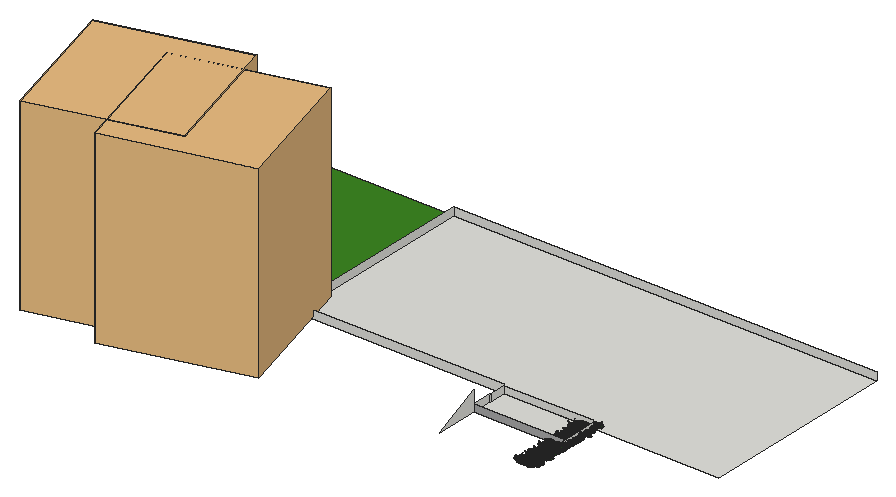
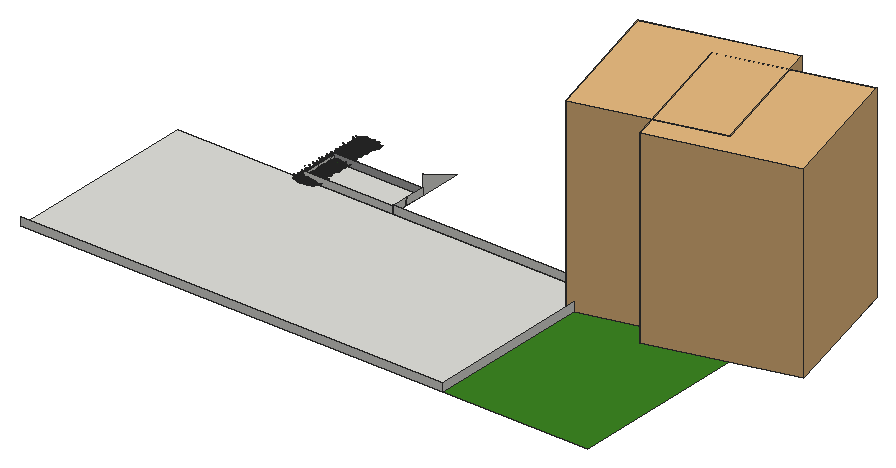
# SketchUp Ruby script. Lengths in inches.
U = 1.inch
M = Sketchup.active_model
def pt(a) = Geom::Point3d.new(a.map { |v| v * U })
def face(e, loops, mat)
  f = e.add_face(loops[0].map { |a| pt(a) })
  loops[1..].each { |l| e.add_face(l.map { |a| pt(a) }).erase! }
  f.material = f.back_material = mat if mat
  f
end
# faces: each face lists its corners as indices into pts; further lists are holes
def faces(e, pts, list, mat = nil) = list.each { |f| face(e, (f[0].is_a?(Array) ? f : [f]).map { |l| l.map { |i| pts[i] } }, mat) }
# xy, xz, yz: faces in a plane at the given z, y or x. An outline is a flat list of corners, or four numbers for a rectangle; further outlines are holes
def ring(l) = l.size == 4 ? [[l[0], l[1]], [l[2], l[1]], [l[2], l[3]], [l[0], l[3]]] : l.each_slice(2).to_a
def flat(e, list, mat, &to3) = list.each { |f| face(e, (f[0].is_a?(Array) ? f : [f]).map { |l| ring(l).map { |u, v| to3.(u, v) } }, mat) }
def xy(e, z, list, mat = nil) = flat(e, list, mat) { |x, y| [x, y, z] }
def xz(e, y, list, mat = nil) = flat(e, list, mat) { |x, z| [x, y, z] }
def yz(e, x, list, mat = nil) = flat(e, list, mat) { |y, z| [x, y, z] }
def lines(e, pts, list) = list.each { |a, b| e.add_line(pt(pts[a]), pt(pts[b])) }
# prism: a flat outline (further loops are holes) pulled along v
def prism(e, loops, v, mat = nil)
  f = face(e, loops, mat); d = Geom::Vector3d.new(v.map { |x| x * U })
  f.pushpull(f.normal.samedirection?(d) ? d.length : -d.length)
end
def box(e, o, s, mat = nil) = prism(e, [[o, [o[0] + s[0], o[1], o[2]], [o[0] + s[0], o[1] + s[1], o[2]], [o[0], o[1] + s[1], o[2]]]], [0, 0, s[2]], mat)
def at(x, y, z, deg = 0) = Geom::Transformation.translation(pt([x, y, z])) * Geom::Transformation.rotation(ORIGIN, Z_AXIS, deg.degrees)
def axes(o, x, y, z) = Geom::Transformation.new([*x, 0, *y, 0, *z, 0, *pt(o).to_a, 1])
def part(name) = M.definitions.add(name)
# library, detail: a bought-in or finely detailed component or shape, given as its bounding box
def library(name, o, s) = part(name).tap { |d| box(d.entities, o, s) }
def detail(e, o, s) = box(e.add_group.entities, o, s)
def put(e, d, t, mat = nil) = e.add_instance(d, t).tap { |i| i.material = mat if mat }
def group(e, t, mat = nil) = e.add_group.tap { |g| g.transformation = t; g.material = mat if mat }.entities
root = M.entities
M.materials.add("Material82").color = [68, 110, 58]
M.materials.add("Material83").color = [48, 90, 38]
M.materials.add("Material84").color = [68, 110, 48]
M.materials.add("Material85").color = [48, 90, 48]
M.materials.add("Material86").color = [58, 110, 58]
M.materials.add("Material87").color = [58, 90, 38]
M.materials.add("Material88").color = [68, 100, 58]
M.materials.add("Material89").color = [48, 100, 38]
M.materials.add("[Color M01]").color = [60, 133, 34]
M.materials.add("[Color M03]1").color = [170, 170, 170]
c1 = library("Palm tree",[-4.09,-4.52,0],[193.52,193.51,258.93])
c2 = part("Palm+Tree")
put(c2.entities,c1,at(25.51,-21.81,0,15))
c3 = library("Group\#612",[0,0,0],[32.91,53.52,103.45])
c4 = part("grass00")
p = [[-0.6875,0.15,0],[-0.56,0.08,5.52],[-0.04,0.03,2.76],[0.48,-0.02,0],[0.35,-0.02,5.52],[-0.1,-0.14,5.52],
  [-0.12,0.65,8.37],[-0.42,0.65,8.37]]
faces(c4.entities,p,[[0,1,2,3],[3,2,4],[1,5,2],[5,4,2],[1,6,5],[4,5,6],[7,6,1]])
c5 = part("Group16\#1")
put(c5.entities,c4,axes([1.44,-0.61,-0.01],[0.05352,0.12609,0],[-0.10704,0.04543,0.07239],[0.06664,-0.02828,0.11628]),"Material85")
put(c5.entities,c4,axes([0.76,-0.15,-0.01],[0.04676,0.24062,0],[-0.23162,0.04501,0.06642],[0.0652,-0.01267,0.23595]),"Material82")
put(c5.entities,c4,axes([0.79,0.01,-0.01],[-0.00606,0.34651,0],[-0.34381,-0.00602,0.0432],[0.04319,0.00076,0.34386]))
put(c5.entities,c4,axes([1,0.23,-0.01],[-0.07192,0.31144,0],[-0.28722,-0.06632,0.1236],[0.12043,0.02781,0.29478]),"Material84")
put(c5.entities,c4,axes([1.66,0.77,-0.01],[-0.13828,0.29651,0],[-0.21551,-0.1005,0.22471],[0.20365,0.09498,0.23779]),"Material89")
put(c5.entities,c4,axes([0.6875,0.52,-0.01],[-0.18126,0.24051,0],[-0.22746,-0.17142,0.09788],[0.07817,0.05891,0.28481]),"Material84")
put(c5.entities,c4,axes([0.68,0.78,-0.01],[-0.215,0.18688,0],[-0.12385,-0.14248,0.21334],[0.13995,0.16101,0.18878]),"Material82")
put(c5.entities,c4,axes([0.56,1,-0.01],[-0.13756,0.07624,0],[-0.06159,-0.11112,0.0927],[0.04494,0.08108,0.12705]),"Material84")
put(c5.entities,c4,axes([0.2,0.64,-0.01],[-0.23729,0.07254,0],[-0.05711,-0.18681,0.153],[0.04473,0.14632,0.19535]),"Material89")
put(c5.entities,c4,axes([0.0625,0.72,-0.01],[-0.28874,0.02525,0],[-0.02179,-0.24916,0.14647],[0.01276,0.14591,0.25012]),"Material82")
put(c5.entities,c4,axes([-0.08,0.62,-0.01],[-0.34089,-0.04187,0],[0.03255,-0.26504,0.216],[-0.02633,0.21439,0.26703]),"Material89")
put(c5.entities,c4,axes([-0.34,0.98,-0.01],[-0.14314,-0.0493,0],[0.04397,-0.12769,0.06843],[-0.02228,0.0647,0.13505]),"Material89")
put(c5.entities,c4,axes([-0.87,1.45,-0.01],[-0.23488,-0.14114,0],[0.13761,-0.22901,0.06087],[-0.03135,0.05217,0.26717]))
put(c5.entities,c4,axes([-0.72,0.77,-0.01],[-0.14208,-0.13251,0],[0.07209,-0.0773,0.16301],[-0.11118,0.11922,0.1057]),"Material89")
put(c5.entities,c4,axes([-0.62,0.43,-0.01],[-0.14845,-0.21203,0],[0.18654,-0.13061,0.12304],[-0.10079,0.07057,0.22772]),"Material82")
put(c5.entities,c4,axes([-0.68,0.29,-0.01],[-0.13639,-0.32136,0],[0.31723,-0.13464,0.05579],[-0.05136,0.0218,0.34462]),"Material83")
put(c5.entities,c4,axes([-0.64,0.125,-0.01],[-0.0458,-0.23569,0],[0.22124,-0.043,0.08276],[-0.08124,0.01579,0.22538]),"Material86")
put(c5.entities,c4,axes([-1.6,-0.03,-0.01],[0.00576,-0.32897,0],[0.27526,0.00482,0.18018],[-0.18015,-0.00315,0.2753]),"Material84")
put(c5.entities,c4,axes([-1.36,-0.31,-0.01],[0.05718,-0.24765,0],[0.18172,0.04196,0.17267],[-0.16825,-0.03885,0.1865]),"Material89")
put(c5.entities,c4,axes([-1.54,-0.72,-0.01],[0.06537,-0.14017,0],[0.13555,0.06321,0.03939],[-0.0357,-0.01665,0.14956]))
put(c5.entities,c4,axes([-1.19,-0.9,-0.01],[0.09597,-0.12735,0],[0.11214,0.08451,0.07557],[-0.06035,-0.04548,0.14042]),"Material88")
put(c5.entities,c4,axes([-0.47,-0.54,-0.01],[0.11588,-0.10072,0],[0.0618,0.0711,0.12124],[-0.07953,-0.0915,0.0942]))
put(c5.entities,c4,axes([-0.47,-0.84,-0.01],[0.11927,-0.0661,0],[0.06603,0.11913,0.00646],[-0.00313,-0.00565,0.13621]),"Material84")
put(c5.entities,c4,axes([-0.38,-1.24,-0.01],[0.28037,-0.08571,0],[0.0618,0.20215,0.20315],[-0.05939,-0.19428,0.21139]),"Material88")
put(c5.entities,c4,axes([-0.06,-0.66,-0.01],[0.22719,-0.01987,0],[0.01247,0.14255,0.17758],[-0.01547,-0.17691,0.1431]),"Material87")
put(c5.entities,c4,axes([0.11,-0.89,-0.01],[0.14882,0.01828,0],[-0.01058,0.08611,0.12229],[0.01491,-0.12138,0.08676]),"Material85")
put(c5.entities,c4,axes([0.25,-0.72,-0.01],[0.20481,0.07053,0],[-0.06206,0.18022,0.10291],[0.03351,-0.0973,0.1906]),"Material85")
put(c5.entities,c4,axes([0.85,-1.42,-0.01],[0.16481,0.09904,0],[-0.09472,0.15762,0.05616],[0.02893,-0.04814,0.18389]),"Material84")
put(c5.entities,c4,axes([1.01,-1.09,-0.01],[0.21858,0.20385,0],[-0.17495,0.1876,0.15339],[0.10462,-0.11218,0.25652]),"Material89")
put(c5.entities,c4,axes([1.01,-0.71,-0.01],[0.08733,0.12473,0],[-0.06445,0.04512,0.13037],[0.1068,-0.07477,0.07867]),"Material85")
c6 = part("Group15\#1")
put(c6.entities,c5,at(0,0,0))
c7 = part("3darcstudiotree_grass00\#1")
put(c7.entities,c6,at(0,0,0))
xy(root,-29.74,[[1163.9375,932.5,1248,932.62],[1534.38,994.94,1657.0625,1046.93],[1248,1046.93,1830.75,1318.18]])
xy(root,-29.74,[[1048.3125,932.62,1248,1318.18]],"[Color M01]")
xz(root,994.94,[[1534.38,-29.74,1657.0625,-19.8125]],"[Color M03]1")
xz(root,1046.93,[[1248,-29.74,1256.88,-19.8125],[1256.88,-29.74,1534.38,-18.36],[1534.38,-29.74,1657.0625,-19.8125]])
xz(root,1318.18,[[1248,-29.74,1830.75,-18.36]])
yz(root,1248,[[935.62,-29.74,994.94,-2.1875,994.94,-29.74],[994.94,-29.74,1046.93,-19.8125],[1046.93,-29.74,1318.18,-18.36]])
yz(root,1534.38,[[935.62,-29.74,994.94,-29.74,994.94,-2.1875],[994.94,-29.74,1022.06,-19.8125],[1022.06,-29.74,1023.55,-19.8125],[1023.55,-29.74,1046.93,-19.8125]])
yz(root,1657.0625,[[994.94,-29.74,1000.12,-23.22],[1000.12,-29.74,1022.06,-23.22],[1022.06,-29.74,1046.93,-23.22]])
put(root,c2,at(990.42,891.52,-29.74))
put(root,c3,axes([1115.36,894.49,-29.74],[1.13014,0.75656,0],[-0.75656,1.13014,0],[0,0,1.36]))
put(root,c2,at(1097.35,885.71,-29.74))
put(root,c7,axes([1644.74,1010.04,-29.74],[-3.06097,-0.5879,0],[1.66705,-1.34995,-0.03924],[0.1162,-0.0941,1.93013]))
put(root,c7,axes([1645.43,958.21,-29.74],[-1.33725,-1.41841,0],[4.13991,-0.60704,-0.02925],[0.14115,-0.0207,1.7044]))
put(root,c7,axes([1645.47,946.84,-29.74],[-4.40805,-0.66258,0],[1.20213,-1.24385,-0.04688],[0.1049,-0.10854,1.58936]))
put(root,c7,axes([1645.59,948.47,-29.74],[-4.593,-0.45536,0],[0.84159,-1.32024,-0.02201],[0.02791,-0.04378,1.34565]))
put(root,c7,axes([1644.84,997.65,-29.74],[2.83648,-1.2359,0],[3.15131,1.12486,-0.01132],[0.04822,0.01721,1.83032]))
put(root,c7,axes([1645.85,983.19,-29.74],[-1.4633,-1.68853,0],[3.81957,-0.51482,-0.03013],[0.1448,-0.01952,1.53631]))
put(root,c7,axes([1645.82,1031.95,-29.74],[0.43217,-1.5656,0],[4.20709,0.18062,-0.01362],[0.0661,0.00284,1.54899]))
put(root,c7,axes([1645.35,1035.85,-29.74],[-3.35215,0.96429,0],[-2.54913,-1.37823,-0.03459],[-0.11585,-0.06264,1.84283]))
put(root,c7,axes([1644.58,940.12,-29.74],[3.65261,0,0],[0,1.44049,0],[0,0,1]))
put(root,c7,axes([1646.37,1042.6,-29.74],[-1.52778,-1.4368,0],[3.26203,-0.53947,-0.00949],[0.054,-0.00893,1.63563]))
put(root,c7,axes([1645.32,1044.86,-29.74],[-2.50316,1.24796,0],[-3.26881,-1.01974,-0.0328],[-0.10917,-0.03406,1.32564]))
put(root,c7,axes([1646.31,1014.65,-29.74],[-4.03652,-0.16228,0],[0.44348,-1.71564,-0.03002],[0.01485,-0.05745,1.59842]))
put(root,c7,axes([1644.8125,982.15,-29.74],[3.25905,0.69762,0],[-2.04099,1.48295,-0.01651],[-0.04447,0.03231,1.81134]))
put(root,c7,axes([1645.59,960.26,-29.74],[-1.85538,1.37845,0],[-3.32658,-0.69639,-0.02935],[-0.1215,-0.02544,1.32321]))
put(root,c7,axes([1645.55,1051.48,-29.74],[-1.47744,1.354,0],[-3.50661,-0.5951,-0.01574],[-0.08407,-0.01427,1.66349]))
put(root,c7,axes([1646,1019.44,-29.74],[2.89762,-1.1399,0],[2.43274,0.96179,-0.0036],[0.01556,0.00615,1.5794]))
put(root,c7,axes([1645.48,992.45,-29.74],[-2.16254,1.46376,0],[-3.92939,-0.90288,-0.00219],[-0.00913,-0.0021,1.64693]))
put(root,c7,axes([1645.21,1037.79,-29.74],[3.10066,0.47843,0],[-1.67535,1.68868,-0.03882],[-0.06401,0.06452,1.55956]))
put(root,c7,axes([1645.64,951.63,-29.74],[3.24585,-0.20669,0],[0.57348,1.40067,-0.03713],[0.03058,0.07468,1.39317]))
put(root,c7,axes([1646.22,1048.56,-29.74],[-2.59394,1.01102,0],[-3.072,-1.22583,-0.01852],[-0.05979,-0.02386,1.50457]))
put(root,c7,axes([1645.92,1001.8,-29.74],[3.9501,-0.3019,0],[0.82816,1.68526,-0.01483],[0.01308,0.02661,1.51152]))
put(root,c7,axes([1646.01,979.3,-29.74],[3.32132,-0.19382,0],[0.6507,1.73421,-0.00326],[0.00271,0.00722,1.88794]))
put(root,c7,axes([1645.62,1023.55,-29.74],[3.35543,0.83331,0],[-2.02345,1.2672,-0.03908],[-0.13338,0.08353,1.82303]))
put(root,c7,axes([1645.9,942.22,-29.74],[1.50682,1.6341,0],[-3.24176,0.46492,-0.03897],[-0.21712,0.03114,1.53286]))
put(root,c7,axes([1646.35,1007.71,-29.74],[2.855,1.42821,0],[-2.79418,0.86872,-0.04305],[-0.19263,0.05989,1.51958]))
put(root,c7,axes([1647.98,986.04,-29.74],[-4.71763,0.13616,0],[-0.3116,-1.67918,-0.0067],[-0.002,-0.01078,1.30916]))
put(root,c7,axes([1647.88,992.48,-29.74],[0.36596,-1.66077,0],[4.11633,0.14107,-0.03115],[0.15736,0.00539,1.5702]))
put(root,c7,axes([1648.43,988.04,-29.74],[1.0844,-1.46677,0],[3.4842,0.40063,-0.01207],[0.07085,0.00815,1.66287]))
put(root,c7,axes([1648.82,1045.3125,-29.74],[-3.58141,-0.41852,0],[1.07572,-1.43168,-0.05017],[0.07746,-0.10309,1.54202]))
put(root,c7,axes([1649.23,1036.04,-29.74],[-2.10821,-1.47996,0],[3.50963,-0.77757,-0.0488],[0.18715,-0.04146,1.32723]))
put(root,c7,axes([1648.66,942.81,-29.74],[2.27608,-1.0007,0],[3.35316,1.18618,-0.03873],[0.1622,0.05738,1.89965]))
put(root,c7,axes([1649.13,972.67,-29.74],[-3.59463,0.44793,0],[-1.16817,-1.45801,-0.02199],[-0.03431,-0.04283,1.50537]))
put(root,c7,axes([1649.11,968.48,-29.74],[2.73821,-1.25836,0],[3.57659,1.21044,-0.00643],[0.02336,0.00791,1.6911]))
put(root,c7,axes([1648.05,1030.12,-29.74],[4.14496,0.31804,0],[-0.83759,1.6978,-0.03864],[-0.04159,0.0843,1.85268]))
put(root,c7,axes([1648.27,998.79,-29.74],[4.22455,0.00563,0],[-0.01154,1.34671,-0.00416],[-0.00007,0.00858,1.3392]))
put(root,c7,axes([1648.23,1001.3125,-29.74],[3.14768,1.20624,0],[-3.13864,1.27383,-0.06236],[-0.23969,0.09728,1.86199]))
put(root,c7,axes([1650.02,1051.8125,-29.74],[-2.67553,-0.98375,0],[2.79136,-1.18074,-0.04642],[0.15585,-0.06593,1.51042]))
put(root,c7,axes([1649.55,1026.87,-29.74],[1.22629,-1.22817,0],[3.78204,0.58732,-0.0431],[0.18193,0.02825,1.38217]))
put(root,c7,axes([1648.42,989.92,-29.74],[-0.387,1.5813,0],[-4.71042,-0.17929,-0.01578],[-0.06068,-0.00231,1.37044]))
put(root,c7,axes([1649.6,1013.93,-29.74],[2.09831,-1.02697,0],[3.53268,1.1226,-0.04335],[0.15343,0.04876,1.54559]))
put(root,c7,axes([1650.22,1043.03,-29.74],[-1.12016,-1.49158,0],[3.32126,-0.38792,-0.01669],[0.11216,-0.0131,1.82011]))
put(root,c7,axes([1649.47,1010.39,-29.74],[-2.72452,1.24598,0],[-3.55259,-1.2082,-0.04683],[-0.18808,-0.06396,1.86493]))
put(root,c7,axes([1648.47,958.07,-29.74],[0.67723,1.39261,0],[-4.43088,0.33513,-0.00068],[-0.00322,0.00024,1.62852]))
put(root,c7,axes([1649.93,976.62,-29.74],[1.58844,-1.66939,0],[3.21642,0.47599,-0.02337],[0.14197,0.02101,1.67088]))
put(root,c7,axes([1650.29,946.1,-29.74],[-3.67612,0.09043,0],[-0.28445,-1.79854,-0.0193],[-0.00469,-0.02963,1.33558]))
put(root,c7,axes([1649.25,944.87,-29.74],[0.19969,1.44757,0],[-3.37153,0.07234,-0.03311],[-0.18886,0.00405,1.44579]))
put(root,c7,axes([1650.57,1040.18,-29.74],[-3.74626,-0.28421,0],[0.67953,-1.39309,-0.01319],[0.01627,-0.03336,1.76124]))
put(root,c7,axes([1648.95,1016.4,-29.74],[3.77194,0.53127,0],[-1.56854,1.73204,-0.02984],[-0.04464,0.0493,1.55474]))
put(root,c7,axes([1650.63,994.86,-29.74],[0.06282,-1.34984,0],[3.50326,0.02536,-0.01436],[0.0861,0.00062,1.57494]))
put(root,c7,axes([1650.59,1012.27,-29.74],[0.71144,-1.32945,0],[4.31841,0.35942,-0.04294],[0.17046,0.01419,1.34209]))
put(root,c7,axes([1649.82,948.1,-29.74],[-2.51102,1.11498,0],[-3.04783,-1.06754,-0.01682],[-0.06435,-0.02254,1.56312]))
put(root,c7,axes([1651.12,1046.51,-29.74],[-4.08051,-0.34509,0],[0.80518,-1.48079,-0.03168],[0.03378,-0.06213,1.46389]))
put(root,c7,axes([1650.74,982,-29.74],[-3.50605,0.34582,0],[-0.87343,-1.37724,-0.00789],[-0.01222,-0.01927,1.7222]))
put(root,c7,axes([1650.87,1019.35,-29.74],[1.7149,-1.22637,0],[3.67075,0.79833,-0.00061],[0.00329,0.00072,1.94394]))
put(root,c7,axes([1649.63,951.68,-29.74],[4.50029,0.14913,0],[-0.32235,1.51291,-0.00911],[-0.00515,0.02417,1.94776]))
put(root,c7,axes([1651.2,1021.36,-29.74],[1.13517,-1.33714,0],[4.08386,0.53922,-0.04023],[0.16123,0.02129,1.36415]))
put(root,c7,axes([1650.28,1025.36,-29.74],[-1.96155,1.42232,0],[-3.86474,-0.82896,-0.01158],[-0.04562,-0.00979,1.47884]))
put(root,c7,axes([1650.86,975.37,-29.74],[-3.11045,1.07931,0],[-2.57078,-1.15227,-0.02195],[-0.09054,-0.04058,1.82186]))
put(root,c7,axes([1651.68,1031.55,-29.74],[-0.47401,-1.83018,0],[3.81106,-0.15352,-0.01024],[0.06486,-0.00261,1.82793]))
put(root,c7,axes([1651.32,980.125,-29.74],[2.67895,-1.42027,0],[3.76202,1.10364,-0.01386],[0.04132,0.01212,1.30579]))
put(root,c7,axes([1651.89,964.375,-29.74],[-4.02887,-0.32689,0],[0.86941,-1.66657,-0.02294],[0.02463,-0.04722,1.72347]))
put(root,c7,axes([1650.9,959.83,-29.74],[3.37179,-0.80655,0],[2.39395,1.55652,-0.03972],[0.09789,0.06365,1.6444]))
put(root,c7,axes([1650.13,983.55,-29.74],[3.19117,1.02249,0],[-2.28557,1.10943,-0.0068],[-0.02189,0.01063,1.38619]))
put(root,c7,axes([1650.21,966.21,-29.74],[0.53207,1.56479,0],[-4.35061,0.23008,-0.0098],[-0.05087,0.00269,1.72283]))
put(root,c7,axes([1650.34,971.08,-29.74],[3.6725,0.99677,0],[-2.44181,1.39924,-0.05897],[-0.19798,0.11345,1.91169]))
put(root,c7,axes([1651.13,997.62,-29.74],[-1.969,1.11609,0],[-3.42444,-0.93961,-0.02835],[-0.10891,-0.02988,1.46355]))
put(root,c7,axes([1650.5,1034.3125,-29.74],[-0.22309,1.29668,0],[-4.38525,-0.11734,-0.00038],[-0.00168,-0.00004,1.44006]))
put(root,c7,axes([1651.63,954.59,-29.74],[-3.28336,1.15138,0],[-2.69769,-1.19648,-0.01814],[-0.06877,-0.0305,1.73642]))
put(root,c7,axes([1650.81,1037.56,-29.74],[2.78968,1.01154,0],[-2.64,1.13236,-0.04265],[-0.18761,0.08047,1.90027]))
put(root,c7,axes([1651.11,1023,-29.74],[-2.22727,1.60419,0],[-4.12877,-0.89155,-0.00813],[-0.02667,-0.00576,1.31962]))
put(root,c7,axes([1651.45,1007.45,-29.74],[-2.60888,1.40075,0],[-3.4553,-1.0009,-0.02364],[-0.11495,-0.0333,1.93862]))
put(root,c7,axes([1651.83,1006.35,-29.74],[3.43972,-1.19732,0],[3.07284,1.37298,-0.00351],[0.01073,0.00479,1.60808]))
put(root,c7,axes([1651.76,962.37,-29.74],[-2.75837,1.17724,0],[-3.35186,-1.22148,-0.01856],[-0.07358,-0.02681,1.84646]))
put(root,c7,axes([1651.85,1004.03,-29.74],[2.57433,-1.10368,0],[3.03991,1.10279,-0.05921],[0.27011,0.09799,1.91907]))
put(root,c7,axes([1651.38,940.17,-29.74],[4.03336,-0.1179,0],[0.28483,1.51556,-0.02045],[0.00943,0.05018,1.8024]))
put(root,c7,axes([1651.86,1049.3125,-29.74],[-2.1063,1.53486,0],[-3.86767,-0.82549,-0.04902],[-0.23106,-0.04932,1.76654]))
put(root,c7,axes([1653.77,1023.5,-29.74],[-1.00872,-1.50256,0],[3.76018,-0.39261,-0.00114],[0.00668,-0.0007,1.77079]))
put(root,c7,axes([1651.85,953.76,-29.74],[1.54692,1.35045,0],[-3.5946,0.6404,-0.01637],[-0.06936,0.01236,1.37485]))
put(root,c7,axes([1653.42,987.9,-29.74],[-1.02138,-1.60708,0],[3.36091,-0.33222,-0.0349],[0.24018,-0.02374,1.84282]))
put(root,c7,axes([1654.0625,1010.12,-29.74],[-4.39065,-0.68044,0],[1.48247,-1.48779,-0.03326],[0.06181,-0.06203,1.54402]))
put(root,c7,axes([1654.05,1024.88,-29.74],[-4.44259,0.07323,0],[-0.15396,-1.45277,-0.02048],[-0.00618,-0.05831,1.99696]))
put(root,c7,axes([1653.56,1020.67,-29.74],[-2.76199,0.84111,0],[-2.40625,-1.22891,-0.02049],[-0.06035,-0.03082,1.42185]))
put(root,c7,axes([1654.45,948.87,-29.74],[-4.39876,-0.08421,0],[0.22064,-1.79246,-0.01036],[0.00206,-0.01674,1.39846]))
put(root,c7,axes([1654.0625,1036.34,-29.74],[2.13524,-1.29449,0],[3.0122,0.77275,-0.01966],[0.10051,0.02579,1.64285]))
put(root,c7,axes([1654.78,975.56,-29.74],[-2.27298,-1.15312,0],[2.90139,-0.88948,-0.04864],[0.26323,-0.0807,1.88819]))
put(root,c7,axes([1654.77,957.29,-29.74],[-0.27323,-1.39515,0],[4.04907,-0.12333,-0.04603],[0.24308,-0.0074,1.61216]))
put(root,c7,axes([1654.25,995.35,-29.74],[-3.30373,1.03648,0],[-2.84639,-1.41107,-0.00639],[-0.01873,-0.00928,1.6128]))
put(root,c7,axes([1655.25,977.95,-29.74],[-4.23108,-0.20575,0],[0.45076,-1.44167,-0.03319],[0.02288,-0.07317,1.55524]))
put(root,c7,axes([1654.69,1044.59,-29.74],[-2.75278,0.82906,0],[-2.65464,-1.37089,-0.0597],[-0.21369,-0.11035,1.93343]))
put(root,c7,axes([1654.25,1049.82,-29.74],[-1.7142,1.30326,0],[-3.68982,-0.75483,-0.04385],[-0.17675,-0.03616,1.41492]))
put(root,c7,axes([1654.75,1037.99,-29.74],[-2.52665,1.52426,0],[-3.1276,-0.80632,-0.05029],[-0.29899,-0.07708,1.98932]))
put(root,c7,axes([1655.07,1033.74,-29.74],[1.00905,-1.48256,0],[4.12419,0.43657,-0.05256],[0.2523,0.02671,1.59089]))
put(root,c7,axes([1655.5625,991.87,-29.74],[-1.34868,-1.52366,0],[4.27,-0.58784,-0.05387],[0.21958,-0.03023,1.46363]))
put(root,c7,axes([1655.51,1042.67,-29.74],[-0.81771,-1.39799,0],[3.86882,-0.35195,-0.03351],[0.1754,-0.01596,1.59864]))
put(root,c7,axes([1654.16,1003.57,-29.74],[4.22079,-0.16227,0],[0.44484,1.79962,-0.00515],[0.00263,0.01065,1.80879]))
put(root,c7,axes([1654.23,966.15,-29.74],[3.56541,-0.13016,0],[0.37676,1.60514,-0.05657],[0.02546,0.10845,1.49576]))
put(root,c7,axes([1655.04,968.125,-29.74],[-3.05652,0.90078,0],[-1.97442,-1.04198,-0.01872],[-0.07362,-0.03885,1.62421]))
put(root,c7,axes([1655.23,945.04,-29.74],[-3.18956,0.31713,0],[-1.10467,-1.728,-0.01943],[-0.01876,-0.02934,1.33771]))
put(root,c7,axes([1655.79,981.1,-29.74],[-3.13974,-0.75675,0],[2.02292,-1.30536,-0.04274],[0.1274,-0.08221,1.66217]))
put(root,c7,axes([1655.91,985.7,-29.74],[-4.11825,0.06325,0],[-0.12995,-1.31605,-0.00954],[-0.0021,-0.02124,1.41434]))
put(root,c7,axes([1655.03,983.48,-29.74],[-0.62058,1.51993,0],[-3.60511,-0.22893,-0.03829],[-0.23497,-0.01492,1.70109]))
put(root,c7,axes([1656.28,1000.55,-29.74],[-4.16244,-0.15093,0],[0.36502,-1.56574,-0.01686],[0.00714,-0.03063,1.38194]))
put(root,c7,axes([1656.4375,972.77,-29.74],[-0.89443,-1.66932,0],[4.23179,-0.35265,-0.02196],[0.11928,-0.00994,1.79942]))
put(root,c7,axes([1654.65,963.48,-29.74],[2.80483,0.78712,0],[-2.29694,1.27299,-0.00585],[-0.01927,0.01068,1.68777]))
put(root,c7,axes([1656.08,951.6875,-29.74],[1.02165,-1.42104,0],[3.23224,0.36142,-0.01712],[0.09227,0.01032,1.41054]))
put(root,c7,axes([1654.96,1017.22,-29.74],[-0.6643,1.32662,0],[-4.47997,-0.3489,-0.01512],[-0.08059,-0.00628,1.85999]))
put(root,c7,axes([1656.52,1008.36,-29.74],[0.943,-1.41783,0],[3.80413,0.39351,-0.01105],[0.05525,0.00572,1.52421]))
put(root,c7,axes([1656.84,962.71,-29.74],[-4.34806,-0.2749,0],[0.62437,-1.53594,-0.05495],[0.04724,-0.1162,1.60563]))
put(root,c7,axes([1655.08,999.22,-29.74],[0.93193,1.68006,0],[-3.63506,0.3136,-0.00261],[-0.01526,0.00132,1.6704]))
put(root,c7,axes([1655.07,1032.11,-29.74],[2.55431,1.01117,0],[-3.10398,1.2195,-0.03194],[-0.09397,0.03692,1.36388]))
put(root,c7,axes([1656.48,996.35,-29.74],[1.68936,-1.29831,0],[3.68445,0.74564,-0.0206],[0.10358,0.02096,1.75423]))
put(root,c7,axes([1656.7,970.65,-29.74],[0.80832,-1.39105,0],[3.86121,0.34896,-0.01662],[0.09893,0.00894,1.81323]))
put(root,c7,axes([1655.51,960.375,-29.74],[1.77276,1.31188,0],[-3.2596,0.68507,-0.05193],[-0.30681,0.06448,1.85357]))
put(root,c7,axes([1657.16,1014.65,-29.74],[-3.93808,-0.75827,0],[2.05575,-1.66052,-0.06565],[0.13947,-0.11266,1.70067]))
put(root,c7,axes([1657.36,1051.76,-29.74],[-1.23898,-1.77649,0],[4.18164,-0.45359,-0.02011],[0.11729,-0.01272,1.9663]))
put(root,c7,axes([1655.55,1018.35,-29.74],[-0.07538,1.68656,0],[-4.43832,-0.03085,-0.00958],[-0.0427,-0.0003,1.48335]))
put(root,c7,axes([1657.0625,978.6,-29.74],[0.5287,-1.47174,0],[3.5141,0.19634,-0.02485],[0.18259,0.0102,1.97391]))
put(root,c7,axes([1655.93,1039.76,-29.74],[4.04964,0.85012,0],[-2.04869,1.51784,-0.02998],[-0.08539,0.06326,1.98098]))
put(root,c7,axes([1656.39,1006.2,-29.74],[0.31598,1.50106,0],[-3.48689,0.11416,-0.00998],[-0.05116,0.00168,1.34846]))
put(root,c7,axes([1656.95,941.81,-29.74],[3.14916,-0.41283,0],[1.21857,1.44573,-0.00205],[0.00401,0.00476,1.79239]))
put(root,c7,axes([1657.21,1030.27,-29.74],[3.02082,-1.15648,0],[2.42176,0.98385,-0.02978],[0.11407,0.04634,1.43312]))
put(root,c7,axes([1657.03,946.47,-29.74],[-1.68906,1.71794,0],[-3.99186,-0.61041,-0.03012],[-0.15949,-0.02439,1.82227]))
